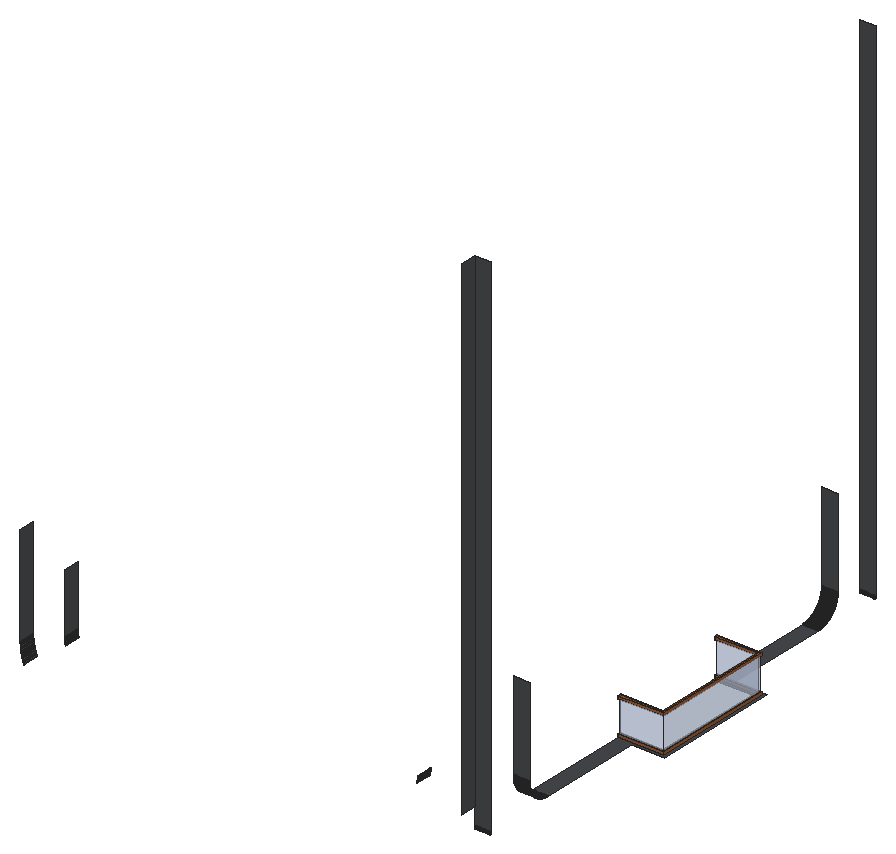
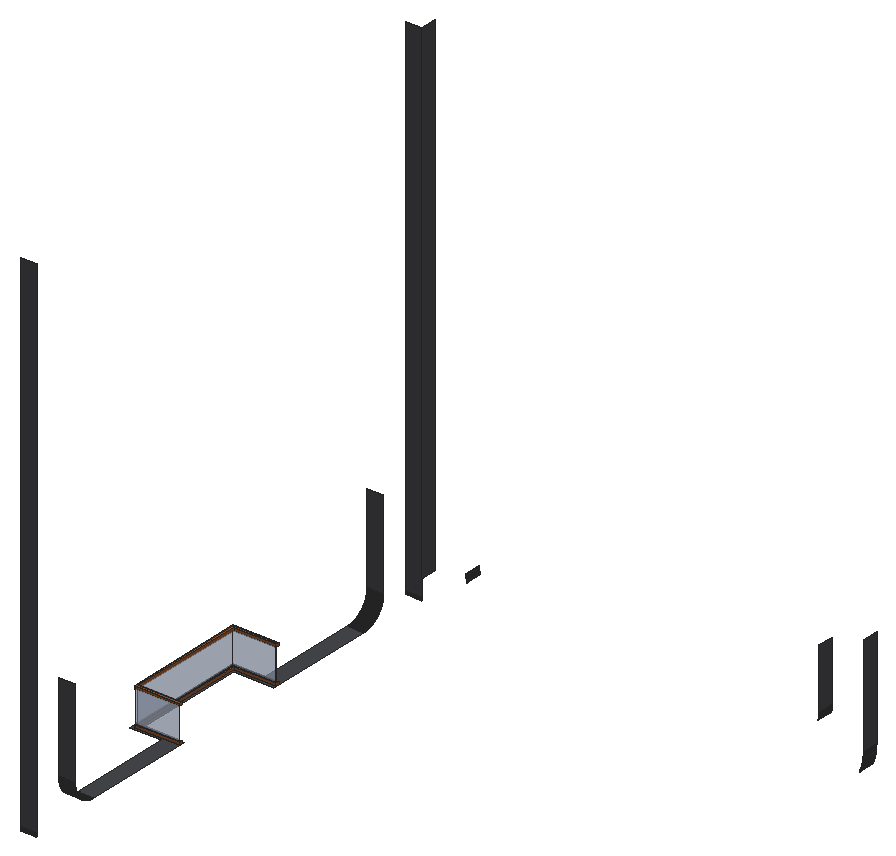
# SketchUp Ruby script. Lengths in inches.
U = 1.inch
M = Sketchup.active_model
def pt(a) = Geom::Point3d.new(a.map { |v| v * U })
def face(e, loops, mat)
  f = e.add_face(loops[0].map { |a| pt(a) })
  loops[1..].each { |l| e.add_face(l.map { |a| pt(a) }).erase! }
  f.material = f.back_material = mat if mat
  f
end
# faces: each face lists its corners as indices into pts; further lists are holes
def faces(e, pts, list, mat = nil) = list.each { |f| face(e, (f[0].is_a?(Array) ? f : [f]).map { |l| l.map { |i| pts[i] } }, mat) }
# xy, xz, yz: faces in a plane at the given z, y or x. An outline is a flat list of corners, or four numbers for a rectangle; further outlines are holes
def ring(l) = l.size == 4 ? [[l[0], l[1]], [l[2], l[1]], [l[2], l[3]], [l[0], l[3]]] : l.each_slice(2).to_a
def flat(e, list, mat, &to3) = list.each { |f| face(e, (f[0].is_a?(Array) ? f : [f]).map { |l| ring(l).map { |u, v| to3.(u, v) } }, mat) }
def xy(e, z, list, mat = nil) = flat(e, list, mat) { |x, y| [x, y, z] }
def xz(e, y, list, mat = nil) = flat(e, list, mat) { |x, z| [x, y, z] }
def yz(e, x, list, mat = nil) = flat(e, list, mat) { |y, z| [x, y, z] }
def lines(e, pts, list) = list.each { |a, b| e.add_line(pt(pts[a]), pt(pts[b])) }
# prism: a flat outline (further loops are holes) pulled along v
def prism(e, loops, v, mat = nil)
  f = face(e, loops, mat); d = Geom::Vector3d.new(v.map { |x| x * U })
  f.pushpull(f.normal.samedirection?(d) ? d.length : -d.length)
end
def box(e, o, s, mat = nil) = prism(e, [[o, [o[0] + s[0], o[1], o[2]], [o[0] + s[0], o[1] + s[1], o[2]], [o[0], o[1] + s[1], o[2]]]], [0, 0, s[2]], mat)
def at(x, y, z, deg = 0) = Geom::Transformation.translation(pt([x, y, z])) * Geom::Transformation.rotation(ORIGIN, Z_AXIS, deg.degrees)
def axes(o, x, y, z) = Geom::Transformation.new([*x, 0, *y, 0, *z, 0, *pt(o).to_a, 1])
def part(name) = M.definitions.add(name)
# library, detail: a bought-in or finely detailed component or shape, given as its bounding box
def library(name, o, s) = part(name).tap { |d| box(d.entities, o, s) }
def detail(e, o, s) = box(e.add_group.entities, o, s)
def put(e, d, t, mat = nil) = e.add_instance(d, t).tap { |i| i.material = mat if mat }
def group(e, t, mat = nil) = e.add_group.tap { |g| g.transformation = t; g.material = mat if mat }.entities
root = M.entities
M.materials.add("1432 AP 8245 TAR ROAD").color = [71, 72, 75]
M.materials.add("[Translucent Glass Blue]").color = [195, 208, 233]
M.materials["[Translucent Glass Blue]"].alpha = 0.5
M.materials.add("[Wood Cherry Original]").color = [152, 86, 42]
c1 = part("Group\#47")
xy(c1.entities,0,[[0,0,0,2,32,2,32,90,0,90,0,92,34,92,34,0]])
xy(c1.entities,1.75,[[0.75,0.75,33.25,0.75,33.25,91.25,0.75,91.25,0.75,90.75,32.75,90.75,32.75,1.25,0.75,1.25]])
xy(c1.entities,2,[[[0,0,34,0,34,92,0,92,0,90,32,90,32,2,0,2],[0.75,0.75,0.75,1.25,32.75,1.25,32.75,90.75,0.75,90.75,0.75,91.25,33.25,91.25,33.25,0.75]]])
xy(c1.entities,26,[[[0,0,0,2,32,2,32,90,0,90,0,92,34,92,34,0],[0.75,0.75,33.25,0.75,33.25,91.25,0.75,91.25,0.75,90.75,32.75,90.75,32.75,1.25,0.75,1.25]]])
xy(c1.entities,26.25,[[0.75,0.75,0.75,1.25,32.75,1.25,32.75,90.75,0.75,90.75,0.75,91.25,33.25,91.25,33.25,0.75]])
xy(c1.entities,28,[[0,0,34,0,34,92,0,92,0,90,32,90,32,2,0,2]])
xz(c1.entities,0,[[0,0,34,2],[0,26,34,28]])
xz(c1.entities,0.75,[[0.75,1.75,33.25,2],[0.75,26,33.25,26.25]])
xz(c1.entities,1.25,[[0.75,1.75,32.75,2],[0.75,26,32.75,26.25]])
xz(c1.entities,2,[[0,0,32,2],[0,26,32,28]])
xz(c1.entities,90,[[0,0,32,2],[0,26,32,28]])
xz(c1.entities,90.75,[[0.75,1.75,32.75,2],[0.75,26,32.75,26.25]])
xz(c1.entities,91.25,[[0.75,1.75,33.25,2],[0.75,26,33.25,26.25]])
xz(c1.entities,92,[[0,0,34,2],[0,26,34,28]])
yz(c1.entities,0,[[0,0,2,2],[90,0,92,2],[0,26,2,28],[90,26,92,28]])
yz(c1.entities,0.75,[[0.75,1.75,1.25,2],[90.75,1.75,91.25,2],[0.75,26,1.25,26.25],[90.75,26,91.25,26.25]])
yz(c1.entities,32,[[2,0,90,2],[2,26,90,28]])
yz(c1.entities,32.75,[[1.25,1.75,90.75,2],[1.25,26,90.75,26.25]])
yz(c1.entities,33.25,[[0.75,1.75,91.25,2],[0.75,26,91.25,26.25]])
yz(c1.entities,34,[[0,0,92,2],[0,26,92,28]])
g1 = group(c1.entities,at(0.75,0.75,1.75),"[Translucent Glass Blue]")
prism(g1,[[[32,90,0],[0,90,0],[0,90.5,0],[32.5,90.5,0],[32.5,0,0],[0,0,0],[0,0.5,0],[32,0.5,0]]],[0,0,24.5])
xy(root,179.79,[[573,161.13,585,161.37],[573,161.37,585,161.37,585,239.37,609,239.37,609,335.37,585,335.37,585,413.37,573,413.37,573,329.37,603,329.37,603,245.37,573,245.37],[573,413.37,585,413.61]],"1432 AP 8245 TAR ROAD")
xz(root,107.37,[[573,179.51,585,179.79],[573,179.79,585,560.79]],"1432 AP 8245 TAR ROAD")
xz(root,143.37,[[573,197.56,585,197.79],[573,197.79,585,263.79]],"1432 AP 8245 TAR ROAD")
xz(root,431.36,[[573,197.09,585,197.32]],"1432 AP 8245 TAR ROAD")
xz(root,431.37,[[573,197.56,585,197.79],[573,197.79,585,263.79]],"1432 AP 8245 TAR ROAD")
xz(root,467.37,[[573,179.23,585,179.51],[573,179.51,585,179.79],[573,179.79,585,560.79]],"1432 AP 8245 TAR ROAD")
yz(root,243,[[95.37,191.23,107.37,191.51],[95.37,191.51,107.37,191.79],[95.37,191.79,107.37,266.79]],"1432 AP 8245 TAR ROAD")
yz(root,276,[[95.37,206.56,107.37,206.79],[95.37,206.79,107.37,251.79]],"1432 AP 8245 TAR ROAD")
yz(root,276.01,[[95.37,206.09,107.37,206.32]],"1432 AP 8245 TAR ROAD")
yz(root,540,[[95.37,206.39,107.37,206.59],[95.37,206.59,107.37,206.79]],"1432 AP 8245 TAR ROAD")
yz(root,573,[[95.37,191.79,107.37,560.79]],"1432 AP 8245 TAR ROAD")
p = [[573,467.28,177.25],[573,467.3,177.53],[585,467.3,177.53],[585,467.28,177.25],[245.85,107.37,177.75],[245.96,107.37,177.49],
  [245.96,95.37,177.49],[245.85,95.37,177.75],[573,107.42,177.8125],[573,107.44,177.53],[585,107.44,177.53],[585,107.42,177.8125],
  [573,467.32,177.8125],[585,467.32,177.8125],[245.74,107.37,178.02],[245.74,95.37,178.02],[573,107.41,178.1],[585,107.41,178.1],
  [573,467.33,178.1],[585,467.33,178.1],[245.63,107.37,178.28],[245.63,95.37,178.28],[573,107.4,178.38],[585,107.4,178.38],
  [573,467.34,178.38],[585,467.34,178.38],[245.53,107.37,178.54],[245.53,95.37,178.54],[573,107.39,178.66],[585,107.39,178.66],
  [573,467.35,178.66],[585,467.35,178.66],[245.42,107.37,178.8],[245.42,95.37,178.8],[573,107.38,178.94],[585,107.38,178.94],
  [573,467.36,178.94],[585,467.36,178.94],[245.32,107.37,179.07],[245.32,95.37,179.07],[573,107.375,179.23],[585,107.375,179.23],
  [573,467.37,179.23],[585,467.37,179.23],[245.23,107.37,179.33],[245.23,95.37,179.33],[573,107.37,179.51],[585,107.37,179.51],
  [245.13,107.37,179.6],[245.13,95.37,179.6],[245.03,107.37,179.86],[245.03,95.37,179.86],[573,159.96,179.85],[573,159.72,179.87],
  [585,159.72,179.87],[585,159.96,179.85],[573,160.19,179.83],[585,160.19,179.83],[573,160.43,179.82],[585,160.43,179.82],
  [573,160.66,179.81],[585,160.66,179.81],[573,160.9,179.8],[585,160.9,179.8],[573,161.13,179.79],[585,161.13,179.79],
  [573,413.84,179.8],[573,413.61,179.79],[585,413.61,179.79],[585,413.84,179.8],[573,414.08,179.81],[585,414.08,179.81],
  [573,414.3125,179.82],[585,414.3125,179.82],[573,414.55,179.83],[585,414.55,179.83],[573,414.78,179.85],[585,414.78,179.85],
  [573,415.02,179.87],[585,415.02,179.87],[244.94,107.37,180.13],[244.94,95.37,180.13],[573,159.02,179.95],[573,158.79,179.98],
  [585,158.79,179.98],[585,159.02,179.95],[573,159.25,179.92],[585,159.25,179.92],[573,159.49,179.89],[585,159.49,179.89],
  [573,415.25,179.89],[585,415.25,179.89],[573,415.49,179.92],[585,415.49,179.92],[573,415.72,179.95],[585,415.72,179.95],
  [573,415.95,179.98],[585,415.95,179.98],[573,158.55,180.01],[573,158.32,180.05],[585,158.32,180.05],[585,158.55,180.01],
  [573,416.1875,180.01],[585,416.1875,180.01],[573,416.42,180.05],[585,416.42,180.05],[244.85,107.37,180.4],[244.85,95.37,180.4],
  [573,157.86,180.14],[573,157.63,180.19],[585,157.63,180.19],[585,157.86,180.14],[573,158.09,180.09],[585,158.09,180.09],
  [573,416.65,180.09],[585,416.65,180.09],[573,416.88,180.14],[585,416.88,180.14],[573,417.11,180.19],[585,417.11,180.19],
  [573,157.4,180.24],[573,157.17,180.29],[585,157.17,180.29],[585,157.4,180.24],[573,417.34,180.24],[585,417.34,180.24],
  [573,417.57,180.29],[585,417.57,180.29],[573,156.9375,180.35],[573,156.71,180.41],[585,156.71,180.41],[585,156.9375,180.35],
  [573,417.8,180.35],[585,417.8,180.35],[573,418.03,180.41],[585,418.03,180.41],[244.76,107.37,180.67],[244.76,95.37,180.67],
  [573,156.48,180.47],[585,156.48,180.47],[573,418.26,180.47],[585,418.26,180.47],[573,156.26,180.53],[573,156.03,180.6],
  [585,156.03,180.6],[585,156.26,180.53],[573,418.48,180.53],[585,418.48,180.53],[573,418.71,180.6],[585,418.71,180.6],
  [573,155.81,180.67],[585,155.81,180.67],[573,418.93,180.67],[585,418.93,180.67],[244.68,107.37,180.9375],[244.68,95.37,180.9375],
  [573,155.58,180.75],[573,155.36,180.82],[585,155.36,180.82],[585,155.58,180.75],[573,419.16,180.75],[585,419.16,180.75],
  [573,419.38,180.82],[585,419.38,180.82],[573,155.14,180.9],[585,155.14,180.9],[573,419.6,180.9],[585,419.6,180.9],
  [244.59,107.37,181.21],[244.59,95.37,181.21],[573,154.92,180.99],[585,154.92,180.99],[573,419.82,180.99],[585,419.82,180.99],
  [573,154.7,181.07],[585,154.7,181.07],[573,420.04,181.07],[585,420.04,181.07],[573,154.48,181.16],[585,154.48,181.16],
  [573,420.26,181.16],[585,420.26,181.16],[244.51,107.37,181.48],[244.51,95.37,181.48],[573,154.26,181.25],[585,154.26,181.25],
  [573,420.48,181.25],[585,420.48,181.25],[573,154.05,181.35],[573,153.83,181.45],[585,153.83,181.45],[585,154.05,181.35],
  [573,420.69,181.35],[585,420.69,181.35],[573,420.91,181.45],[585,420.91,181.45],[573,153.62,181.55],[585,153.62,181.55],
  [573,421.12,181.55],[585,421.12,181.55],[244.43,107.37,181.75],[244.43,95.37,181.75],[573,153.41,181.65],[585,153.41,181.65],
  [573,421.33,181.65],[585,421.33,181.65],[573,153.2,181.75],[585,153.2,181.75],[573,421.54,181.75],[585,421.54,181.75],
  [244.35,107.37,182.02],[244.35,95.37,182.02],[573,152.99,181.86],[585,152.99,181.86],[573,421.75,181.86],[585,421.75,181.86],
  [573,152.78,181.97],[585,152.78,181.97],[573,421.96,181.97],[585,421.96,181.97],[244.28,107.37,182.29],[244.28,95.37,182.29],
  [573,152.57,182.09],[585,152.57,182.09],[573,422.17,182.09],[585,422.17,182.09],[573,152.37,182.2],[585,152.37,182.2],
  [573,422.37,182.2],[585,422.37,182.2],[573,152.17,182.32],[585,152.17,182.32],[573,422.57,182.32],[585,422.57,182.32],
  [244.2,107.37,182.57],[244.2,95.37,182.57],[573,151.96,182.44],[585,151.96,182.44],[573,422.77,182.44],[585,422.77,182.44],
  [573,151.76,182.57],[585,151.76,182.57],[573,422.97,182.57],[585,422.97,182.57],[244.13,107.37,182.84],[244.13,95.37,182.84],
  [573,151.57,182.7],[585,151.57,182.7],[573,423.17,182.7],[585,423.17,182.7],[573,151.37,182.83],[585,151.37,182.83],
  [573,423.37,182.83],[585,423.37,182.83],[244.0625,107.37,183.11],[244.0625,95.37,183.11],[573,151.17,182.96],[585,151.17,182.96],
  [573,423.57,182.96],[585,423.57,182.96],[573,150.98,183.09],[585,150.98,183.09],[573,423.76,183.09],[585,423.76,183.09],
  [243.99,107.37,183.39],[243.99,95.37,183.39],[573,150.79,183.23],[585,150.79,183.23],[573,423.95,183.23],[585,423.95,183.23],
  [573,150.6,183.37],[585,150.6,183.37],[573,424.14,183.37],[585,424.14,183.37],[243.93,107.37,183.66],[243.93,95.37,183.66],
  [573,150.41,183.51],[585,150.41,183.51],[573,424.33,183.51],[585,424.33,183.51],[573,150.23,183.66],[585,150.23,183.66],
  [573,424.51,183.66],[585,424.51,183.66],[243.87,107.37,183.9375],[243.87,95.37,183.9375],[573,150.04,183.8],[585,150.04,183.8],
  [573,424.7,183.8],[585,424.7,183.8],[573,149.86,183.95],[585,149.86,183.95],[573,424.88,183.95],[585,424.88,183.95],
  [243.81,107.37,184.22],[243.81,95.37,184.22],[573,149.68,184.1],[585,149.68,184.1],[573,425.06,184.1],[585,425.06,184.1],
  [573,149.5,184.26],[585,149.5,184.26],[573,425.24,184.26],[585,425.24,184.26],[243.75,107.37,184.49],[243.75,95.37,184.49],
  [573,149.33,184.42],[585,149.33,184.42],[573,425.41,184.42],[585,425.41,184.42],[573,149.15,184.57],[585,149.15,184.57],
  [573,425.59,184.57],[585,425.59,184.57],[243.69,107.37,184.77],[243.69,95.37,184.77],[573,148.98,184.74],[585,148.98,184.74],
  [573,425.76,184.74],[585,425.76,184.74],[573,148.81,184.9],[585,148.81,184.9],[573,425.93,184.9],[585,425.93,184.9],
  [243.64,107.37,185.05],[243.64,95.37,185.05],[573,148.64,185.0625],[585,148.64,185.0625],[573,426.1,185.0625],[585,426.1,185.0625],
  [243.59,107.37,185.32],[243.59,95.37,185.32],[573,148.48,185.23],[585,148.48,185.23],[573,426.26,185.23],[585,426.26,185.23],
  [573,148.3125,185.4],[585,148.3125,185.4],[573,426.43,185.4],[585,426.43,185.4],[243.54,107.37,185.6],[243.54,95.37,185.6],
  [573,148.15,185.57],[585,148.15,185.57],[573,426.59,185.57],[585,426.59,185.57],[243.49,107.37,185.88],[243.49,95.37,185.88],
  [573,147.99,185.75],[585,147.99,185.75],[573,426.75,185.75],[585,426.75,185.75],[573,147.84,185.92],[585,147.84,185.92],
  [573,426.9,185.92],[585,426.9,185.92],[243.44,107.37,186.16],[243.44,95.37,186.16],[573,147.68,186.1],[585,147.68,186.1],
  [573,427.06,186.1],[585,427.06,186.1],[573,147.53,186.28],[585,147.53,186.28],[573,427.21,186.28],[585,427.21,186.28],
  [243.4,107.37,186.44],[243.4,95.37,186.44],[573,147.38,186.46],[585,147.38,186.46],[573,427.36,186.46],[585,427.36,186.46],
  [243.36,107.37,186.72],[243.36,95.37,186.72],[573,147.23,186.65],[585,147.23,186.65],[573,427.51,186.65],[585,427.51,186.65],
  [573,147.09,186.83],[585,147.09,186.83],[573,427.65,186.83],[585,427.65,186.83],[243.32,107.37,187],[243.32,95.37,187],
  [573,146.95,187.02],[585,146.95,187.02],[573,427.79,187.02],[585,427.79,187.02],[243.28,107.37,187.28],[243.28,95.37,187.28],
  [573,146.81,187.21],[585,146.81,187.21],[573,427.93,187.21],[585,427.93,187.21],[573,146.67,187.4],[585,146.67,187.4],
  [573,428.07,187.4],[585,428.07,187.4],[243.25,107.37,187.5625],[243.25,95.37,187.5625],[573,146.54,187.6],[585,146.54,187.6],
  [573,428.2,187.6],[585,428.2,187.6],[243.22,107.37,187.84],[243.22,95.37,187.84],[573,146.4,187.79],[585,146.4,187.79],
  [573,428.34,187.79],[585,428.34,187.79],[243.1875,107.37,188.12],[243.1875,95.37,188.12],[573,146.27,187.99],[585,146.27,187.99],
  [573,428.47,187.99],[585,428.47,187.99],[573,146.15,188.1875],[585,146.15,188.1875],[573,428.59,188.1875],[585,428.59,188.1875],
  [243.16,107.37,188.4],[243.16,95.37,188.4],[573,146.02,188.39],[585,146.02,188.39],[573,428.72,188.39],[585,428.72,188.39],
  [243.13,107.37,188.6875],[243.13,95.37,188.6875],[573,145.9,188.59],[585,145.9,188.59],[573,428.84,188.59],[585,428.84,188.59],
  [573,145.78,188.79],[585,145.78,188.79],[573,428.96,188.79],[585,428.96,188.79],[243.11,107.37,188.97],[243.11,95.37,188.97],
  [573,145.67,189],[585,145.67,189],[573,429.07,189],[585,429.07,189],[243.09,107.37,189.25],[243.09,95.37,189.25],
  [573,145.55,189.2],[585,145.55,189.2],[573,429.1875,189.2],[585,429.1875,189.2],[243.07,107.37,189.53],[243.07,95.37,189.53],
  [573,145.44,189.41],[585,145.44,189.41],[573,429.3,189.41],[585,429.3,189.41],[573,145.33,189.62],[585,145.33,189.62],
  [573,429.41,189.62],[585,429.41,189.62],[243.05,107.37,189.8125],[243.05,95.37,189.8125],[573,145.23,189.83],[585,145.23,189.83],
  [573,429.51,189.83],[585,429.51,189.83],[243.04,107.37,190.1],[243.04,95.37,190.1],[573,145.125,190.04],[585,145.125,190.04],
  [573,429.62,190.04],[585,429.62,190.04],[573,145.02,190.26],[585,145.02,190.26],[573,429.72,190.26],[585,429.72,190.26],
  [243.03,107.37,190.38],[243.03,95.37,190.38],[573,144.93,190.47],[585,144.93,190.47],[573,429.8125,190.47],[585,429.8125,190.47],
  [243.02,107.37,190.66],[243.02,95.37,190.66],[573,144.83,190.6875],[585,144.83,190.6875],[573,429.91,190.6875],[585,429.91,190.6875],
  [243.01,107.37,190.94],[243.01,95.37,190.94],[573,144.74,190.9],[585,144.74,190.9],[573,430,190.9],[585,430,190.9],
  [243,107.37,191.23],[243,95.37,191.23],[573,144.65,191.12],[585,144.65,191.12],[573,430.09,191.12],[585,430.09,191.12],
  [573,144.57,191.34],[585,144.57,191.34],[573,430.17,191.34],[585,430.17,191.34],[573,144.48,191.5625],[585,144.48,191.5625],
  [573,430.26,191.5625],[585,430.26,191.5625],[573,144.4,191.78],[585,144.4,191.78],[573,430.34,191.78],[585,430.34,191.78],
  [573,144.33,192.01],[585,144.33,192.01],[573,430.41,192.01],[585,430.41,192.01],[573,144.25,192.23],[585,144.25,192.23],
  [573,430.49,192.23],[585,430.49,192.23],[573,144.18,192.45],[585,144.18,192.45],[573,430.56,192.45],[585,430.56,192.45],
  [573,144.11,192.68],[585,144.11,192.68],[573,430.63,192.68],[585,430.63,192.68],[573,144.05,192.91],[585,144.05,192.91],
  [573,430.69,192.91],[585,430.69,192.91],[573,143.98,193.13],[585,143.98,193.13],[573,430.76,193.13],[585,430.76,193.13],
  [573,143.92,193.36],[585,143.92,193.36],[573,430.82,193.36],[585,430.82,193.36],[573,143.87,193.59],[585,143.87,193.59],
  [573,430.87,193.59],[585,430.87,193.59],[573,143.8125,193.82],[585,143.8125,193.82],[573,430.93,193.82],[585,430.93,193.82],
  [573,143.76,194.05],[585,143.76,194.05],[573,430.98,194.05],[585,430.98,194.05],[573,143.72,194.28],[585,143.72,194.28],
  [573,431.02,194.28],[585,431.02,194.28],[573,143.67,194.51],[585,143.67,194.51],[573,431.07,194.51],[585,431.07,194.51],
  [573,143.63,194.74],[585,143.63,194.74],[573,431.11,194.74],[585,431.11,194.74],[573,143.59,194.98],[585,143.59,194.98],
  [573,431.15,194.98],[585,431.15,194.98],[573,143.56,195.21],[585,143.56,195.21],[573,431.18,195.21],[585,431.18,195.21],
  [573,143.52,195.44],[585,143.52,195.44],[573,431.22,195.44],[585,431.22,195.44],[573,143.49,195.68],[585,143.49,195.68],
  [573,431.25,195.68],[585,431.25,195.68],[573,143.47,195.91],[585,143.47,195.91],[573,431.27,195.91],[585,431.27,195.91],
  [573,143.45,196.15],[585,143.45,196.15],[573,431.29,196.15],[585,431.29,196.15],[573,143.43,196.38],[585,143.43,196.38],
  [573,431.3125,196.38],[585,431.3125,196.38],[573,143.41,196.61],[585,143.41,196.61],[573,431.33,196.61],[585,431.33,196.61],
  [573,143.39,196.85],[585,143.39,196.85],[573,431.35,196.85],[585,431.35,196.85],[573,143.38,197.09],[585,143.38,197.09],
  [573,431.36,197.09],[585,431.36,197.09],[573,143.375,197.32],[585,143.375,197.32],[573,143.37,197.56],[585,143.37,197.56],
  [573,431.37,197.56],[573,431.36,197.32],[585,431.36,197.32],[585,431.37,197.56],[276.88,107.37,201.23],[276.81,107.37,201.45],
  [276.81,95.37,201.45],[276.88,95.37,201.23],[539.18,107.37,201.42],[539.12,107.37,201.23],[539.12,95.37,201.23],[539.18,95.37,201.42],
  [539.24,107.37,201.62],[539.24,95.37,201.62],[276.74,107.37,201.68],[276.74,95.37,201.68],[539.3,107.37,201.81],[539.3,95.37,201.81],
  [276.68,107.37,201.91],[276.68,95.37,201.91],[539.35,107.37,202],[539.35,95.37,202],[276.61,107.37,202.13],[276.61,95.37,202.13],
  [539.4,107.37,202.2],[539.4,95.37,202.2],[276.55,107.37,202.36],[276.55,95.37,202.36],[539.45,107.37,202.39],[539.45,95.37,202.39],
  [276.5,107.37,202.59],[276.5,95.37,202.59],[539.5,107.37,202.59],[539.5,95.37,202.59],[276.44,107.37,202.82],[276.44,95.37,202.82],
  [539.55,107.37,202.79],[539.55,95.37,202.79],[276.39,107.37,203.05],[276.39,95.37,203.05],[539.59,107.37,202.98],[539.59,95.37,202.98],
  [276.35,107.37,203.28],[276.35,95.37,203.28],[539.63,107.37,203.18],[539.63,95.37,203.18],[539.67,107.37,203.38],[539.67,95.37,203.38],
  [276.3,107.37,203.51],[276.3,95.37,203.51],[539.71,107.37,203.58],[539.71,95.37,203.58],[276.26,107.37,203.74],[276.26,95.37,203.74],
  [539.75,107.37,203.78],[539.75,95.37,203.78],[276.22,107.37,203.98],[276.22,95.37,203.98],[539.78,107.37,203.98],[539.78,95.37,203.98],
  [276.1875,107.37,204.21],[276.1875,95.37,204.21],[539.81,107.37,204.18],[539.81,95.37,204.18],[276.15,107.37,204.44],[276.15,95.37,204.44],
  [539.84,107.37,204.375],[539.84,95.37,204.375],[276.125,107.37,204.68],[276.125,95.37,204.68],[539.86,107.37,204.58],[539.86,95.37,204.58],
  [539.89,107.37,204.78],[539.89,95.37,204.78],[276.1,107.37,204.91],[276.1,95.37,204.91],[539.91,107.37,204.98],[539.91,95.37,204.98],
  [276.08,107.37,205.15],[276.08,95.37,205.15],[539.93,107.37,205.18],[539.93,95.37,205.18],[276.06,107.37,205.38],[276.06,95.37,205.38],
  [539.94,107.37,205.38],[539.94,95.37,205.38],[276.04,107.37,205.61],[276.04,95.37,205.61],[539.96,107.37,205.58],[539.96,95.37,205.58],
  [276.02,107.37,205.85],[276.02,95.37,205.85],[539.97,107.37,205.78],[539.97,95.37,205.78],[539.98,107.37,205.98],[539.98,95.37,205.98],
  [276.01,107.37,206.09],[276.01,95.37,206.09],[539.99,107.37,206.1875],[539.99,95.37,206.1875],[540,107.37,206.39],[540,95.37,206.39],
  [276.01,107.37,206.32],[276,107.37,206.56],[276,95.37,206.56],[276.01,95.37,206.32]]
faces(root,p,[[0,1,2,3],[4,5,6,7],[8,9,10,11],[1,12,13,2],[14,4,7,15],[16,8,11,17],[12,18,19,13],[20,14,15,21],
  [22,16,17,23],[18,24,25,19],[26,20,21,27],[28,22,23,29],[24,30,31,25],[32,26,27,33],[34,28,29,35],[30,36,37,31],
  [38,32,33,39],[40,34,35,41],[36,42,43,37],[44,38,39,45],[46,40,41,47],[48,44,45,49],[50,48,49,51],[52,53,54,55],
  [56,52,55,57],[58,56,57,59],[60,58,59,61],[62,60,61,63],[64,62,63,65],[66,67,68,69],[70,66,69,71],[72,70,71,73],
  [74,72,73,75],[76,74,75,77],[78,76,77,79],[80,50,51,81],[82,83,84,85],[86,82,85,87],[88,86,87,89],[53,88,89,54],
  [90,78,79,91],[92,90,91,93],[94,92,93,95],[96,94,95,97],[98,99,100,101],[83,98,101,84],[102,96,97,103],[104,102,103,105],
  [106,80,81,107],[108,109,110,111],[112,108,111,113],[99,112,113,100],[114,104,105,115],[116,114,115,117],[118,116,117,119],[120,121,122,123],
  [109,120,123,110],[124,118,119,125],[126,124,125,127],[128,129,130,131],[121,128,131,122],[132,126,127,133],[134,132,133,135],[136,106,107,137],
  [129,138,139,130],[140,134,135,141],[142,143,144,145],[138,142,145,139],[146,140,141,147],[148,146,147,149],[143,150,151,144],[152,148,149,153],
  [154,136,137,155],[156,157,158,159],[150,156,159,151],[160,152,153,161],[162,160,161,163],[157,164,165,158],[166,162,163,167],[168,154,155,169],
  [164,170,171,165],[172,166,167,173],[170,174,175,171],[176,172,173,177],[174,178,179,175],[180,176,177,181],[182,168,169,183],[178,184,185,179],
  [186,180,181,187],[188,189,190,191],[184,188,191,185],[192,186,187,193],[194,192,193,195],[189,196,197,190],[198,194,195,199],[200,182,183,201],
  [196,202,203,197],[204,198,199,205],[202,206,207,203],[208,204,205,209],[210,200,201,211],[206,212,213,207],[214,208,209,215],[212,216,217,213],
  [218,214,215,219],[220,210,211,221],[216,222,223,217],[224,218,219,225],[222,226,227,223],[228,224,225,229],[226,230,231,227],[232,228,229,233],
  [234,220,221,235],[230,236,237,231],[238,232,233,239],[236,240,241,237],[242,238,239,243],[244,234,235,245],[240,246,247,241],[248,242,243,249],
  [246,250,251,247],[252,248,249,253],[254,244,245,255],[250,256,257,251],[258,252,253,259],[256,260,261,257],[262,258,259,263],[264,254,255,265],
  [260,266,267,261],[268,262,263,269],[266,270,271,267],[272,268,269,273],[274,264,265,275],[270,276,277,271],[278,272,273,279],[276,280,281,277],
  [282,278,279,283],[284,274,275,285],[280,286,287,281],[288,282,283,289],[286,290,291,287],[292,288,289,293],[294,284,285,295],[290,296,297,291],
  [298,292,293,299],[296,300,301,297],[302,298,299,303],[304,294,295,305],[300,306,307,301],[308,302,303,309],[306,310,311,307],[312,308,309,313],
  [314,304,305,315],[310,316,317,311],[318,312,313,319],[316,320,321,317],[322,318,319,323],[324,314,315,325],[320,326,327,321],[328,322,323,329],
  [330,324,325,331],[326,332,333,327],[334,328,329,335],[332,336,337,333],[338,334,335,339],[340,330,331,341],[336,342,343,337],[344,338,339,345],
  [346,340,341,347],[342,348,349,343],[350,344,345,351],[348,352,353,349],[354,350,351,355],[356,346,347,357],[352,358,359,353],[360,354,355,361],
  [358,362,363,359],[364,360,361,365],[366,356,357,367],[362,368,369,363],[370,364,365,371],[372,366,367,373],[368,374,375,369],[376,370,371,377],
  [374,378,379,375],[380,376,377,381],[382,372,373,383],[378,384,385,379],[386,380,381,387],[388,382,383,389],[384,390,391,385],[392,386,387,393],
  [390,394,395,391],[396,392,393,397],[398,388,389,399],[394,400,401,395],[402,396,397,403],[404,398,399,405],[400,406,407,401],[408,402,403,409],
  [410,404,405,411],[406,412,413,407],[414,408,409,415],[412,416,417,413],[418,414,415,419],[420,410,411,421],[416,422,423,417],[424,418,419,425],
  [426,420,421,427],[422,428,429,423],[430,424,425,431],[428,432,433,429],[434,430,431,435],[436,426,427,437],[432,438,439,433],[440,434,435,441],
  [442,436,437,443],[438,444,445,439],[446,440,441,447],[448,442,443,449],[444,450,451,445],[452,446,447,453],[450,454,455,451],[456,452,453,457],
  [458,448,449,459],[454,460,461,455],[462,456,457,463],[464,458,459,465],[460,466,467,461],[468,462,463,469],[466,470,471,467],[472,468,469,473],
  [474,464,465,475],[470,476,477,471],[478,472,473,479],[480,474,475,481],[476,482,483,477],[484,478,479,485],[486,480,481,487],[482,488,489,483],
  [490,484,485,491],[492,486,487,493],[488,494,495,489],[496,490,491,497],[494,498,499,495],[500,496,497,501],[498,502,503,499],[504,500,501,505],
  [502,506,507,503],[508,504,505,509],[506,510,511,507],[512,508,509,513],[510,514,515,511],[516,512,513,517],[514,518,519,515],[520,516,517,521],
  [518,522,523,519],[524,520,521,525],[522,526,527,523],[528,524,525,529],[526,530,531,527],[532,528,529,533],[530,534,535,531],[536,532,533,537],
  [534,538,539,535],[540,536,537,541],[538,542,543,539],[544,540,541,545],[542,546,547,543],[548,544,545,549],[546,550,551,547],[552,548,549,553],
  [550,554,555,551],[556,552,553,557],[554,558,559,555],[560,556,557,561],[558,562,563,559],[564,560,561,565],[562,566,567,563],[568,564,565,569],
  [566,570,571,567],[572,568,569,573],[570,574,575,571],[576,572,573,577],[574,578,579,575],[580,576,577,581],[578,582,583,579],[584,580,581,585],
  [582,586,587,583],[588,584,585,589],[586,590,591,587],[592,588,589,593],[590,594,595,591],[596,592,593,597],[594,598,599,595],[600,596,597,601],
  [598,602,603,599],[602,604,605,603],[606,607,608,609],[610,611,612,613],[614,615,616,617],[618,614,617,619],[611,620,621,612],[622,618,619,623],
  [620,624,625,621],[626,622,623,627],[624,628,629,625],[630,626,627,631],[628,632,633,629],[634,630,631,635],[632,636,637,633],[638,634,635,639],
  [636,640,641,637],[642,638,639,643],[640,644,645,641],[646,642,643,647],[644,648,649,645],[650,646,647,651],[652,650,651,653],[648,654,655,649],
  [656,652,653,657],[654,658,659,655],[660,656,657,661],[658,662,663,659],[664,660,661,665],[662,666,667,663],[668,664,665,669],[666,670,671,667],
  [672,668,669,673],[670,674,675,671],[676,672,673,677],[678,676,677,679],[674,680,681,675],[682,678,679,683],[680,684,685,681],[686,682,683,687],
  [684,688,689,685],[690,686,687,691],[688,692,693,689],[694,690,691,695],[692,696,697,693],[698,694,695,699],[700,698,699,701],[696,702,703,697],
  [704,700,701,705],[706,704,705,707],[708,709,710,711]],"1432 AP 8245 TAR ROAD")
put(root,c1,at(573,241.37,179.79),"[Wood Cherry Original]")
